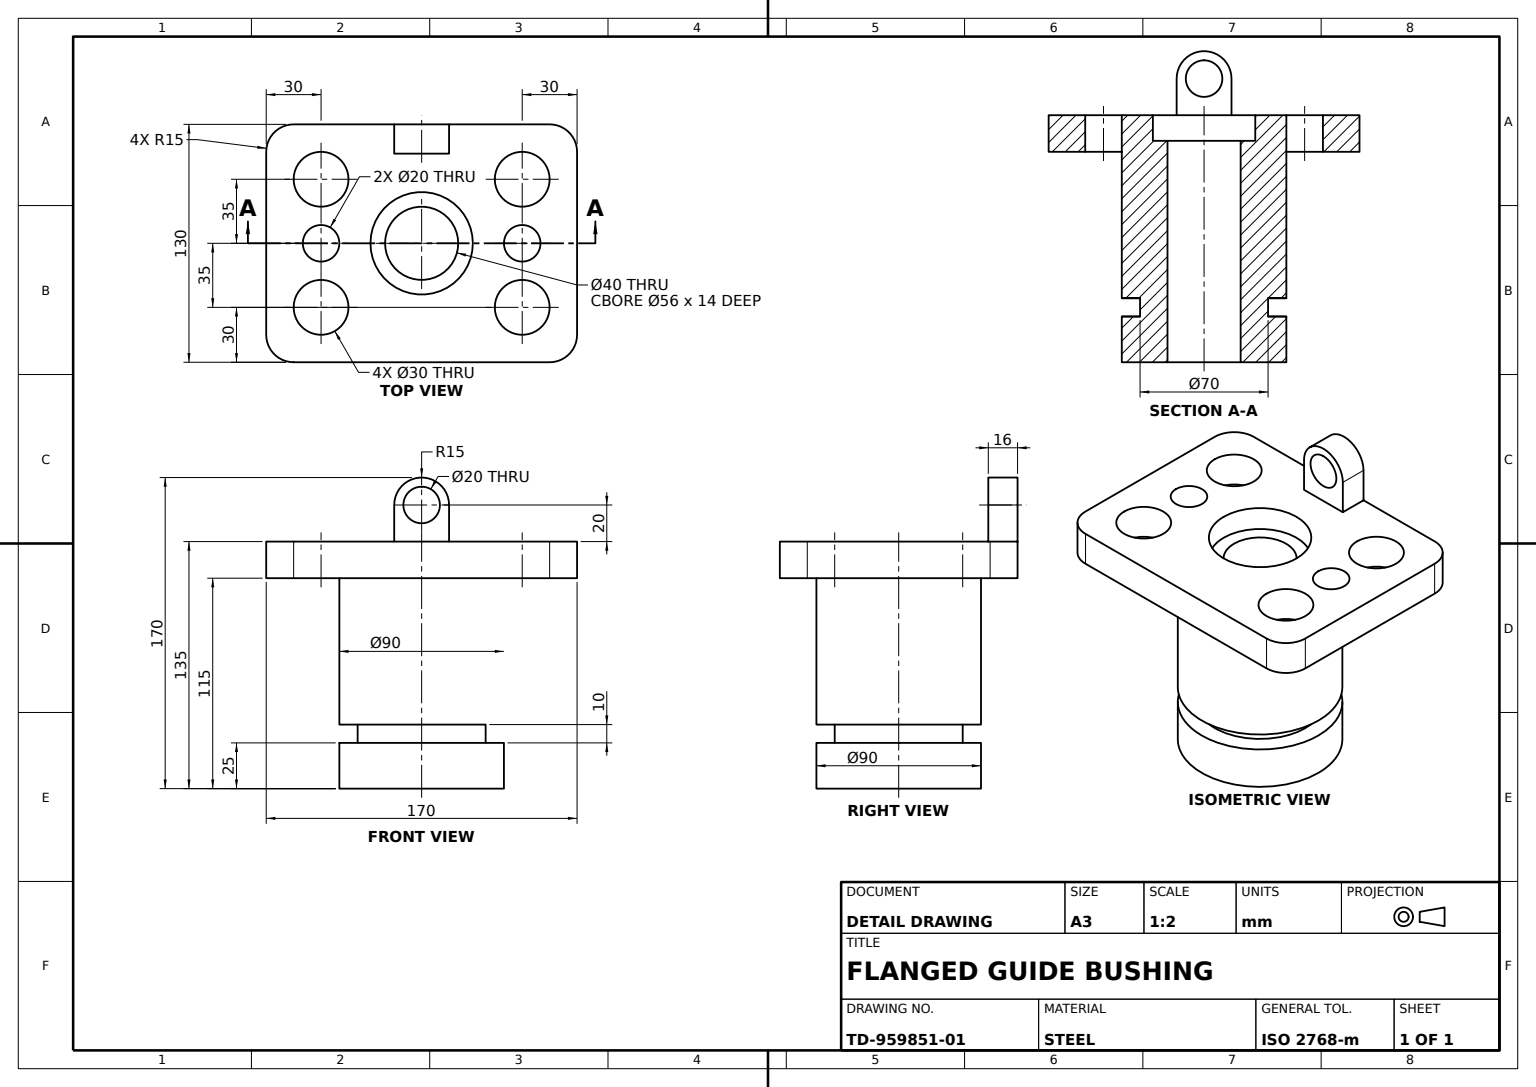
ISO-10303-21;
HEADER;
FILE_DESCRIPTION((''),'2;1');
FILE_NAME('','',(''),(''),'','','');
FILE_SCHEMA(('AUTOMOTIVE_DESIGN'));
ENDSEC;
DATA;
#1=APPLICATION_CONTEXT('');
#2=PRODUCT_CONTEXT('',#1,'mechanical');
#3=PRODUCT('','','',(#2));
#4=PRODUCT_DEFINITION_FORMATION('','',#3);
#5=PRODUCT_DEFINITION_CONTEXT('',#1,'design');
#6=PRODUCT_DEFINITION('','',#4,#5);
#7=PRODUCT_DEFINITION_SHAPE('','',#6);
#8=(LENGTH_UNIT()NAMED_UNIT(*)SI_UNIT(.MILLI.,.METRE.));
#9=(NAMED_UNIT(*)PLANE_ANGLE_UNIT()SI_UNIT($,.RADIAN.));
#10=(NAMED_UNIT(*)SI_UNIT($,.STERADIAN.)SOLID_ANGLE_UNIT());
#11=UNCERTAINTY_MEASURE_WITH_UNIT(LENGTH_MEASURE(0.005),#8,'distance_accuracy_value','');
#12=(GEOMETRIC_REPRESENTATION_CONTEXT(3)GLOBAL_UNCERTAINTY_ASSIGNED_CONTEXT((#11))GLOBAL_UNIT_ASSIGNED_CONTEXT((#8,#9,#10))REPRESENTATION_CONTEXT('',''));
#13=CARTESIAN_POINT('',(-35.,0.,35.));
#14=VERTEX_POINT('',#13);
#15=CARTESIAN_POINT('',(0.,0.,35.));
#16=DIRECTION('',(0.,0.,-1.));
#17=DIRECTION('',(-1.,0.,0.));
#18=AXIS2_PLACEMENT_3D('',#15,#16,#17);
#19=CIRCLE('',#18,35.);
#20=EDGE_CURVE('',#14,#14,#19,.F.);
#21=ORIENTED_EDGE('',*,*,#20,.T.);
#22=EDGE_LOOP('',(#21));
#23=FACE_BOUND('',#22,.T.);
#24=CARTESIAN_POINT('',(-45.,0.,35.));
#25=VERTEX_POINT('',#24);
#26=CIRCLE('',#18,45.);
#27=EDGE_CURVE('',#25,#25,#26,.F.);
#28=ORIENTED_EDGE('',*,*,#27,.F.);
#29=EDGE_LOOP('',(#28));
#30=FACE_BOUND('',#29,.T.);
#31=CARTESIAN_POINT('',(0.,35.,35.));
#32=AXIS2_PLACEMENT_3D('',#31,#16,#17);
#33=PLANE('',#32);
#34=ADVANCED_FACE('',(#23,#30),#33,.T.);
#35=CARTESIAN_POINT('',(45.,0.,115.));
#36=VERTEX_POINT('',#35);
#37=CARTESIAN_POINT('',(55.,0.,115.));
#38=DIRECTION('',(0.,0.,1.));
#39=DIRECTION('',(1.,0.,0.));
#40=AXIS2_PLACEMENT_3D('',#37,#38,#39);
#41=CIRCLE('',#40,10.);
#42=EDGE_CURVE('',#36,#36,#41,.T.);
#43=ORIENTED_EDGE('',*,*,#42,.F.);
#44=EDGE_LOOP('',(#43));
#45=FACE_BOUND('',#44,.T.);
#46=CARTESIAN_POINT('',(45.,0.,135.));
#47=VERTEX_POINT('',#46);
#48=CARTESIAN_POINT('',(55.,0.,135.));
#49=AXIS2_PLACEMENT_3D('',#48,#16,#17);
#50=CIRCLE('',#49,10.);
#51=EDGE_CURVE('',#47,#47,#50,.T.);
#52=ORIENTED_EDGE('',*,*,#51,.F.);
#53=EDGE_LOOP('',(#52));
#54=FACE_BOUND('',#53,.T.);
#55=CYLINDRICAL_SURFACE('',#49,10.);
#56=ADVANCED_FACE('',(#45,#54),#55,.F.);
#57=CARTESIAN_POINT('',(-70.,65.,135.));
#58=VERTEX_POINT('',#57);
#59=CARTESIAN_POINT('',(-85.,50.,135.));
#60=VERTEX_POINT('',#59);
#61=CARTESIAN_POINT('',(-70.,50.,135.));
#62=AXIS2_PLACEMENT_3D('',#61,#38,#39);
#63=CIRCLE('',#62,15.);
#64=EDGE_CURVE('',#58,#60,#63,.T.);
#65=ORIENTED_EDGE('',*,*,#64,.F.);
#66=CARTESIAN_POINT('',(-70.,65.,115.));
#67=VERTEX_POINT('',#66);
#68=VECTOR('',#16,1000.);
#69=LINE('',#57,#68);
#70=EDGE_CURVE('',#67,#58,#69,.F.);
#71=ORIENTED_EDGE('',*,*,#70,.F.);
#72=CARTESIAN_POINT('',(-85.,50.,115.));
#73=VERTEX_POINT('',#72);
#74=CARTESIAN_POINT('',(-70.,50.,115.));
#75=AXIS2_PLACEMENT_3D('',#74,#38,#39);
#76=CIRCLE('',#75,15.);
#77=EDGE_CURVE('',#73,#67,#76,.F.);
#78=ORIENTED_EDGE('',*,*,#77,.F.);
#79=LINE('',#59,#68);
#80=EDGE_CURVE('',#60,#73,#79,.T.);
#81=ORIENTED_EDGE('',*,*,#80,.F.);
#82=EDGE_LOOP('',(#65,#71,#78,#81));
#83=FACE_BOUND('',#82,.T.);
#84=AXIS2_PLACEMENT_3D('',#61,#16,#17);
#85=CYLINDRICAL_SURFACE('',#84,15.);
#86=ADVANCED_FACE('',(#83),#85,.T.);
#87=CARTESIAN_POINT('',(15.,49.,155.));
#88=VERTEX_POINT('',#87);
#89=CARTESIAN_POINT('',(-15.,49.,155.));
#90=VERTEX_POINT('',#89);
#91=CARTESIAN_POINT('',(0.,49.,155.));
#92=DIRECTION('',(0.,-1.,0.));
#93=AXIS2_PLACEMENT_3D('',#91,#92,#39);
#94=CIRCLE('',#93,15.);
#95=EDGE_CURVE('',#88,#90,#94,.T.);
#96=ORIENTED_EDGE('',*,*,#95,.F.);
#97=CARTESIAN_POINT('',(15.,65.,155.));
#98=VERTEX_POINT('',#97);
#99=VECTOR('',#92,1000.);
#100=LINE('',#97,#99);
#101=EDGE_CURVE('',#98,#88,#100,.T.);
#102=ORIENTED_EDGE('',*,*,#101,.F.);
#103=CARTESIAN_POINT('',(-15.,65.,155.));
#104=VERTEX_POINT('',#103);
#105=CARTESIAN_POINT('',(0.,65.,155.));
#106=AXIS2_PLACEMENT_3D('',#105,#92,#39);
#107=CIRCLE('',#106,15.);
#108=EDGE_CURVE('',#98,#104,#107,.T.);
#109=ORIENTED_EDGE('',*,*,#108,.T.);
#110=LINE('',#103,#99);
#111=EDGE_CURVE('',#104,#90,#110,.T.);
#112=ORIENTED_EDGE('',*,*,#111,.T.);
#113=EDGE_LOOP('',(#96,#102,#109,#112));
#114=FACE_BOUND('',#113,.T.);
#115=AXIS2_PLACEMENT_3D('',#105,#92,#16);
#116=CYLINDRICAL_SURFACE('',#115,15.);
#117=ADVANCED_FACE('',(#114),#116,.T.);
#118=CARTESIAN_POINT('',(-70.,-65.,115.));
#119=VERTEX_POINT('',#118);
#120=CARTESIAN_POINT('',(-85.,-50.,115.));
#121=VERTEX_POINT('',#120);
#122=CARTESIAN_POINT('',(-70.,-50.,115.));
#123=AXIS2_PLACEMENT_3D('',#122,#38,#39);
#124=CIRCLE('',#123,15.);
#125=EDGE_CURVE('',#119,#121,#124,.F.);
#126=ORIENTED_EDGE('',*,*,#125,.F.);
#127=CARTESIAN_POINT('',(-70.,-65.,135.));
#128=VERTEX_POINT('',#127);
#129=LINE('',#127,#68);
#130=EDGE_CURVE('',#128,#119,#129,.T.);
#131=ORIENTED_EDGE('',*,*,#130,.F.);
#132=CARTESIAN_POINT('',(-85.,-50.,135.));
#133=VERTEX_POINT('',#132);
#134=CARTESIAN_POINT('',(-70.,-50.,135.));
#135=AXIS2_PLACEMENT_3D('',#134,#38,#39);
#136=CIRCLE('',#135,15.);
#137=EDGE_CURVE('',#133,#128,#136,.T.);
#138=ORIENTED_EDGE('',*,*,#137,.F.);
#139=LINE('',#132,#68);
#140=EDGE_CURVE('',#121,#133,#139,.F.);
#141=ORIENTED_EDGE('',*,*,#140,.F.);
#142=EDGE_LOOP('',(#126,#131,#138,#141));
#143=FACE_BOUND('',#142,.T.);
#144=AXIS2_PLACEMENT_3D('',#134,#16,#17);
#145=CYLINDRICAL_SURFACE('',#144,15.);
#146=ADVANCED_FACE('',(#143),#145,.T.);
#147=CARTESIAN_POINT('',(70.,-65.,135.));
#148=VERTEX_POINT('',#147);
#149=CARTESIAN_POINT('',(-85.,-65.,135.));
#150=VECTOR('',#39,1000.);
#151=LINE('',#149,#150);
#152=EDGE_CURVE('',#128,#148,#151,.T.);
#153=ORIENTED_EDGE('',*,*,#152,.F.);
#154=ORIENTED_EDGE('',*,*,#130,.T.);
#155=CARTESIAN_POINT('',(70.,-65.,115.));
#156=VERTEX_POINT('',#155);
#157=CARTESIAN_POINT('',(-85.,-65.,115.));
#158=LINE('',#157,#150);
#159=EDGE_CURVE('',#119,#156,#158,.T.);
#160=ORIENTED_EDGE('',*,*,#159,.T.);
#161=LINE('',#147,#68);
#162=EDGE_CURVE('',#156,#148,#161,.F.);
#163=ORIENTED_EDGE('',*,*,#162,.T.);
#164=EDGE_LOOP('',(#153,#154,#160,#163));
#165=FACE_BOUND('',#164,.T.);
#166=DIRECTION('',(0.,1.,0.));
#167=AXIS2_PLACEMENT_3D('',#149,#166,#38);
#168=PLANE('',#167);
#169=ADVANCED_FACE('',(#165),#168,.F.);
#170=ORIENTED_EDGE('',*,*,#80,.T.);
#171=CARTESIAN_POINT('',(-85.,65.,115.));
#172=LINE('',#171,#99);
#173=EDGE_CURVE('',#73,#121,#172,.T.);
#174=ORIENTED_EDGE('',*,*,#173,.T.);
#175=ORIENTED_EDGE('',*,*,#140,.T.);
#176=CARTESIAN_POINT('',(-85.,65.,135.));
#177=LINE('',#176,#99);
#178=EDGE_CURVE('',#60,#133,#177,.T.);
#179=ORIENTED_EDGE('',*,*,#178,.F.);
#180=EDGE_LOOP('',(#170,#174,#175,#179));
#181=FACE_BOUND('',#180,.T.);
#182=AXIS2_PLACEMENT_3D('',#176,#39,#16);
#183=PLANE('',#182);
#184=ADVANCED_FACE('',(#181),#183,.F.);
#185=CARTESIAN_POINT('',(-35.,0.,25.));
#186=VERTEX_POINT('',#185);
#187=CARTESIAN_POINT('',(0.,0.,25.));
#188=AXIS2_PLACEMENT_3D('',#187,#16,#17);
#189=CIRCLE('',#188,35.);
#190=EDGE_CURVE('',#186,#186,#189,.F.);
#191=ORIENTED_EDGE('',*,*,#190,.F.);
#192=EDGE_LOOP('',(#191));
#193=FACE_BOUND('',#192,.T.);
#194=CARTESIAN_POINT('',(45.,0.,25.));
#195=VERTEX_POINT('',#194);
#196=AXIS2_PLACEMENT_3D('',#187,#38,#39);
#197=CIRCLE('',#196,45.);
#198=EDGE_CURVE('',#195,#195,#197,.F.);
#199=ORIENTED_EDGE('',*,*,#198,.F.);
#200=EDGE_LOOP('',(#199));
#201=FACE_BOUND('',#200,.T.);
#202=CARTESIAN_POINT('',(0.,45.521823,25.));
#203=AXIS2_PLACEMENT_3D('',#202,#38,#39);
#204=PLANE('',#203);
#205=ADVANCED_FACE('',(#193,#201),#204,.T.);
#206=ORIENTED_EDGE('',*,*,#20,.F.);
#207=EDGE_LOOP('',(#206));
#208=FACE_BOUND('',#207,.T.);
#209=ORIENTED_EDGE('',*,*,#190,.T.);
#210=EDGE_LOOP('',(#209));
#211=FACE_BOUND('',#210,.T.);
#212=CARTESIAN_POINT('',(0.,0.,0.));
#213=AXIS2_PLACEMENT_3D('',#212,#16,#17);
#214=CYLINDRICAL_SURFACE('',#213,35.);
#215=ADVANCED_FACE('',(#208,#211),#214,.T.);
#216=CARTESIAN_POINT('',(-45.,0.,115.));
#217=VERTEX_POINT('',#216);
#218=CARTESIAN_POINT('',(0.,0.,115.));
#219=AXIS2_PLACEMENT_3D('',#218,#38,#39);
#220=CIRCLE('',#219,45.);
#221=EDGE_CURVE('',#36,#217,#220,.T.);
#222=ORIENTED_EDGE('',*,*,#221,.F.);
#223=EDGE_CURVE('',#217,#36,#220,.T.);
#224=ORIENTED_EDGE('',*,*,#223,.F.);
#225=EDGE_LOOP('',(#222,#224));
#226=FACE_BOUND('',#225,.T.);
#227=ORIENTED_EDGE('',*,*,#27,.T.);
#228=EDGE_LOOP('',(#227));
#229=FACE_BOUND('',#228,.T.);
#230=CARTESIAN_POINT('',(0.,0.,135.));
#231=AXIS2_PLACEMENT_3D('',#230,#16,#17);
#232=CYLINDRICAL_SURFACE('',#231,45.);
#233=ADVANCED_FACE('',(#226,#229),#232,.T.);
#234=CARTESIAN_POINT('',(-20.,0.,0.));
#235=VERTEX_POINT('',#234);
#236=CIRCLE('',#213,20.);
#237=EDGE_CURVE('',#235,#235,#236,.T.);
#238=ORIENTED_EDGE('',*,*,#237,.T.);
#239=EDGE_LOOP('',(#238));
#240=FACE_BOUND('',#239,.T.);
#241=CARTESIAN_POINT('',(-20.,0.,121.));
#242=VERTEX_POINT('',#241);
#243=CARTESIAN_POINT('',(0.,0.,121.));
#244=AXIS2_PLACEMENT_3D('',#243,#16,#17);
#245=CIRCLE('',#244,20.);
#246=EDGE_CURVE('',#242,#242,#245,.F.);
#247=ORIENTED_EDGE('',*,*,#246,.T.);
#248=EDGE_LOOP('',(#247));
#249=FACE_BOUND('',#248,.T.);
#250=CARTESIAN_POINT('',(0.,0.,-71.66739));
#251=AXIS2_PLACEMENT_3D('',#250,#16,#17);
#252=CYLINDRICAL_SURFACE('',#251,20.);
#253=ADVANCED_FACE('',(#240,#249),#252,.F.);
#254=CARTESIAN_POINT('',(-15.,65.,135.));
#255=VERTEX_POINT('',#254);
#256=CARTESIAN_POINT('',(-15.,49.,135.));
#257=VERTEX_POINT('',#256);
#258=CARTESIAN_POINT('',(-15.,0.,135.));
#259=LINE('',#258,#99);
#260=EDGE_CURVE('',#255,#257,#259,.T.);
#261=ORIENTED_EDGE('',*,*,#260,.T.);
#262=LINE('',#89,#68);
#263=EDGE_CURVE('',#90,#257,#262,.T.);
#264=ORIENTED_EDGE('',*,*,#263,.F.);
#265=ORIENTED_EDGE('',*,*,#111,.F.);
#266=LINE('',#103,#68);
#267=EDGE_CURVE('',#104,#255,#266,.T.);
#268=ORIENTED_EDGE('',*,*,#267,.T.);
#269=EDGE_LOOP('',(#261,#264,#265,#268));
#270=FACE_BOUND('',#269,.T.);
#271=AXIS2_PLACEMENT_3D('',#103,#17,#38);
#272=PLANE('',#271);
#273=ADVANCED_FACE('',(#270),#272,.T.);
#274=CARTESIAN_POINT('',(15.,49.,135.));
#275=VERTEX_POINT('',#274);
#276=CARTESIAN_POINT('',(15.,49.,122.516247));
#277=VECTOR('',#38,1000.);
#278=LINE('',#276,#277);
#279=EDGE_CURVE('',#275,#88,#278,.T.);
#280=ORIENTED_EDGE('',*,*,#279,.F.);
#281=CARTESIAN_POINT('',(15.,65.,135.));
#282=VERTEX_POINT('',#281);
#283=CARTESIAN_POINT('',(15.,0.,135.));
#284=VECTOR('',#166,1000.);
#285=LINE('',#283,#284);
#286=EDGE_CURVE('',#275,#282,#285,.T.);
#287=ORIENTED_EDGE('',*,*,#286,.T.);
#288=CARTESIAN_POINT('',(15.,65.,122.516247));
#289=LINE('',#288,#277);
#290=EDGE_CURVE('',#282,#98,#289,.T.);
#291=ORIENTED_EDGE('',*,*,#290,.T.);
#292=ORIENTED_EDGE('',*,*,#101,.T.);
#293=EDGE_LOOP('',(#280,#287,#291,#292));
#294=FACE_BOUND('',#293,.T.);
#295=AXIS2_PLACEMENT_3D('',#288,#39,#16);
#296=PLANE('',#295);
#297=ADVANCED_FACE('',(#294),#296,.T.);
#298=CARTESIAN_POINT('',(45.,0.,0.));
#299=VERTEX_POINT('',#298);
#300=AXIS2_PLACEMENT_3D('',#212,#16,#39);
#301=CIRCLE('',#300,45.);
#302=EDGE_CURVE('',#299,#299,#301,.T.);
#303=ORIENTED_EDGE('',*,*,#302,.T.);
#304=EDGE_LOOP('',(#303));
#305=FACE_BOUND('',#304,.T.);
#306=ORIENTED_EDGE('',*,*,#237,.F.);
#307=EDGE_LOOP('',(#306));
#308=FACE_BOUND('',#307,.T.);
#309=PLANE('',#213);
#310=ADVANCED_FACE('',(#305,#308),#309,.T.);
#311=CARTESIAN_POINT('',(-40.,35.,115.));
#312=VERTEX_POINT('',#311);
#313=CARTESIAN_POINT('',(-55.,35.,115.));
#314=AXIS2_PLACEMENT_3D('',#313,#38,#39);
#315=CIRCLE('',#314,15.);
#316=EDGE_CURVE('',#312,#312,#315,.T.);
#317=ORIENTED_EDGE('',*,*,#316,.T.);
#318=EDGE_LOOP('',(#317));
#319=FACE_BOUND('',#318,.T.);
#320=CARTESIAN_POINT('',(-40.,-35.,115.));
#321=VERTEX_POINT('',#320);
#322=CARTESIAN_POINT('',(-55.,-35.,115.));
#323=AXIS2_PLACEMENT_3D('',#322,#38,#39);
#324=CIRCLE('',#323,15.);
#325=EDGE_CURVE('',#321,#321,#324,.T.);
#326=ORIENTED_EDGE('',*,*,#325,.T.);
#327=EDGE_LOOP('',(#326));
#328=FACE_BOUND('',#327,.T.);
#329=CARTESIAN_POINT('',(70.,35.,115.));
#330=VERTEX_POINT('',#329);
#331=CARTESIAN_POINT('',(55.,35.,115.));
#332=AXIS2_PLACEMENT_3D('',#331,#38,#39);
#333=CIRCLE('',#332,15.);
#334=EDGE_CURVE('',#330,#330,#333,.T.);
#335=ORIENTED_EDGE('',*,*,#334,.T.);
#336=EDGE_LOOP('',(#335));
#337=FACE_BOUND('',#336,.T.);
#338=ORIENTED_EDGE('',*,*,#42,.T.);
#339=ORIENTED_EDGE('',*,*,#221,.T.);
#340=CARTESIAN_POINT('',(-55.,0.,115.));
#341=AXIS2_PLACEMENT_3D('',#340,#38,#39);
#342=CIRCLE('',#341,10.);
#343=EDGE_CURVE('',#217,#217,#342,.T.);
#344=ORIENTED_EDGE('',*,*,#343,.T.);
#345=ORIENTED_EDGE('',*,*,#223,.T.);
#346=EDGE_LOOP('',(#338,#339,#344,#345));
#347=FACE_BOUND('',#346,.T.);
#348=CARTESIAN_POINT('',(70.,65.,115.));
#349=VERTEX_POINT('',#348);
#350=CARTESIAN_POINT('',(85.,50.,115.));
#351=VERTEX_POINT('',#350);
#352=CARTESIAN_POINT('',(70.,50.,115.));
#353=AXIS2_PLACEMENT_3D('',#352,#38,#39);
#354=CIRCLE('',#353,15.);
#355=EDGE_CURVE('',#349,#351,#354,.F.);
#356=ORIENTED_EDGE('',*,*,#355,.T.);
#357=CARTESIAN_POINT('',(85.,-50.,115.));
#358=VERTEX_POINT('',#357);
#359=CARTESIAN_POINT('',(85.,-65.,115.));
#360=LINE('',#359,#284);
#361=EDGE_CURVE('',#358,#351,#360,.T.);
#362=ORIENTED_EDGE('',*,*,#361,.F.);
#363=CARTESIAN_POINT('',(70.,-50.,115.));
#364=AXIS2_PLACEMENT_3D('',#363,#38,#39);
#365=CIRCLE('',#364,15.);
#366=EDGE_CURVE('',#358,#156,#365,.F.);
#367=ORIENTED_EDGE('',*,*,#366,.T.);
#368=ORIENTED_EDGE('',*,*,#159,.F.);
#369=ORIENTED_EDGE('',*,*,#125,.T.);
#370=ORIENTED_EDGE('',*,*,#173,.F.);
#371=ORIENTED_EDGE('',*,*,#77,.T.);
#372=CARTESIAN_POINT('',(85.,65.,115.));
#373=VECTOR('',#17,1000.);
#374=LINE('',#372,#373);
#375=EDGE_CURVE('',#349,#67,#374,.T.);
#376=ORIENTED_EDGE('',*,*,#375,.F.);
#377=EDGE_LOOP('',(#356,#362,#367,#368,#369,#370,#371,#376));
#378=FACE_BOUND('',#377,.T.);
#379=CARTESIAN_POINT('',(70.,-35.,115.));
#380=VERTEX_POINT('',#379);
#381=CARTESIAN_POINT('',(55.,-35.,115.));
#382=AXIS2_PLACEMENT_3D('',#381,#38,#39);
#383=CIRCLE('',#382,15.);
#384=EDGE_CURVE('',#380,#380,#383,.T.);
#385=ORIENTED_EDGE('',*,*,#384,.T.);
#386=EDGE_LOOP('',(#385));
#387=FACE_BOUND('',#386,.T.);
#388=PLANE('',#219);
#389=ADVANCED_FACE('',(#319,#328,#337,#347,#378,#387),#388,.F.);
#390=ORIENTED_EDGE('',*,*,#366,.F.);
#391=CARTESIAN_POINT('',(85.,-50.,135.));
#392=VERTEX_POINT('',#391);
#393=LINE('',#391,#68);
#394=EDGE_CURVE('',#392,#358,#393,.T.);
#395=ORIENTED_EDGE('',*,*,#394,.F.);
#396=CARTESIAN_POINT('',(70.,-50.,135.));
#397=AXIS2_PLACEMENT_3D('',#396,#38,#39);
#398=CIRCLE('',#397,15.);
#399=EDGE_CURVE('',#148,#392,#398,.T.);
#400=ORIENTED_EDGE('',*,*,#399,.F.);
#401=ORIENTED_EDGE('',*,*,#162,.F.);
#402=EDGE_LOOP('',(#390,#395,#400,#401));
#403=FACE_BOUND('',#402,.T.);
#404=AXIS2_PLACEMENT_3D('',#396,#16,#17);
#405=CYLINDRICAL_SURFACE('',#404,15.);
#406=ADVANCED_FACE('',(#403),#405,.T.);
#407=CARTESIAN_POINT('',(0.,49.,165.));
#408=VERTEX_POINT('',#407);
#409=AXIS2_PLACEMENT_3D('',#91,#166,#38);
#410=CIRCLE('',#409,10.);
#411=EDGE_CURVE('',#408,#408,#410,.T.);
#412=ORIENTED_EDGE('',*,*,#411,.T.);
#413=EDGE_LOOP('',(#412));
#414=FACE_BOUND('',#413,.T.);
#415=CARTESIAN_POINT('',(0.,49.,135.));
#416=LINE('',#415,#150);
#417=EDGE_CURVE('',#257,#275,#416,.T.);
#418=ORIENTED_EDGE('',*,*,#417,.T.);
#419=ORIENTED_EDGE('',*,*,#279,.T.);
#420=ORIENTED_EDGE('',*,*,#95,.T.);
#421=ORIENTED_EDGE('',*,*,#263,.T.);
#422=EDGE_LOOP('',(#418,#419,#420,#421));
#423=FACE_BOUND('',#422,.T.);
#424=AXIS2_PLACEMENT_3D('',#91,#92,#16);
#425=PLANE('',#424);
#426=ADVANCED_FACE('',(#414,#423),#425,.T.);
#427=CARTESIAN_POINT('',(85.,50.,135.));
#428=VERTEX_POINT('',#427);
#429=LINE('',#427,#68);
#430=EDGE_CURVE('',#351,#428,#429,.F.);
#431=ORIENTED_EDGE('',*,*,#430,.F.);
#432=ORIENTED_EDGE('',*,*,#355,.F.);
#433=CARTESIAN_POINT('',(70.,65.,135.));
#434=VERTEX_POINT('',#433);
#435=LINE('',#433,#68);
#436=EDGE_CURVE('',#434,#349,#435,.T.);
#437=ORIENTED_EDGE('',*,*,#436,.F.);
#438=CARTESIAN_POINT('',(70.,50.,135.));
#439=AXIS2_PLACEMENT_3D('',#438,#38,#39);
#440=CIRCLE('',#439,15.);
#441=EDGE_CURVE('',#428,#434,#440,.T.);
#442=ORIENTED_EDGE('',*,*,#441,.F.);
#443=EDGE_LOOP('',(#431,#432,#437,#442));
#444=FACE_BOUND('',#443,.T.);
#445=AXIS2_PLACEMENT_3D('',#438,#16,#17);
#446=CYLINDRICAL_SURFACE('',#445,15.);
#447=ADVANCED_FACE('',(#444),#446,.T.);
#448=CARTESIAN_POINT('',(-65.,0.,135.));
#449=VERTEX_POINT('',#448);
#450=CARTESIAN_POINT('',(-55.,0.,135.));
#451=AXIS2_PLACEMENT_3D('',#450,#16,#17);
#452=CIRCLE('',#451,10.);
#453=EDGE_CURVE('',#449,#449,#452,.T.);
#454=ORIENTED_EDGE('',*,*,#453,.F.);
#455=EDGE_LOOP('',(#454));
#456=FACE_BOUND('',#455,.T.);
#457=ORIENTED_EDGE('',*,*,#343,.F.);
#458=EDGE_LOOP('',(#457));
#459=FACE_BOUND('',#458,.T.);
#460=CYLINDRICAL_SURFACE('',#451,10.);
#461=ADVANCED_FACE('',(#456,#459),#460,.F.);
#462=ORIENTED_EDGE('',*,*,#325,.F.);
#463=EDGE_LOOP('',(#462));
#464=FACE_BOUND('',#463,.T.);
#465=CARTESIAN_POINT('',(-70.,-35.,135.));
#466=VERTEX_POINT('',#465);
#467=CARTESIAN_POINT('',(-55.,-35.,135.));
#468=AXIS2_PLACEMENT_3D('',#467,#16,#17);
#469=CIRCLE('',#468,15.);
#470=EDGE_CURVE('',#466,#466,#469,.T.);
#471=ORIENTED_EDGE('',*,*,#470,.F.);
#472=EDGE_LOOP('',(#471));
#473=FACE_BOUND('',#472,.T.);
#474=CYLINDRICAL_SURFACE('',#468,15.);
#475=ADVANCED_FACE('',(#464,#473),#474,.F.);
#476=ORIENTED_EDGE('',*,*,#302,.F.);
#477=EDGE_LOOP('',(#476));
#478=FACE_BOUND('',#477,.T.);
#479=ORIENTED_EDGE('',*,*,#198,.T.);
#480=EDGE_LOOP('',(#479));
#481=FACE_BOUND('',#480,.T.);
#482=ADVANCED_FACE('',(#478,#481),#232,.T.);
#483=ORIENTED_EDGE('',*,*,#51,.T.);
#484=EDGE_LOOP('',(#483));
#485=FACE_BOUND('',#484,.T.);
#486=ORIENTED_EDGE('',*,*,#470,.T.);
#487=EDGE_LOOP('',(#486));
#488=FACE_BOUND('',#487,.T.);
#489=CARTESIAN_POINT('',(40.,-35.,135.));
#490=VERTEX_POINT('',#489);
#491=CARTESIAN_POINT('',(55.,-35.,135.));
#492=AXIS2_PLACEMENT_3D('',#491,#16,#17);
#493=CIRCLE('',#492,15.);
#494=EDGE_CURVE('',#490,#490,#493,.T.);
#495=ORIENTED_EDGE('',*,*,#494,.T.);
#496=EDGE_LOOP('',(#495));
#497=FACE_BOUND('',#496,.T.);
#498=CARTESIAN_POINT('',(-28.,0.,135.));
#499=VERTEX_POINT('',#498);
#500=CIRCLE('',#231,28.);
#501=EDGE_CURVE('',#499,#499,#500,.T.);
#502=ORIENTED_EDGE('',*,*,#501,.T.);
#503=EDGE_LOOP('',(#502));
#504=FACE_BOUND('',#503,.T.);
#505=ORIENTED_EDGE('',*,*,#453,.T.);
#506=EDGE_LOOP('',(#505));
#507=FACE_BOUND('',#506,.T.);
#508=CARTESIAN_POINT('',(40.,35.,135.));
#509=VERTEX_POINT('',#508);
#510=CARTESIAN_POINT('',(55.,35.,135.));
#511=AXIS2_PLACEMENT_3D('',#510,#16,#17);
#512=CIRCLE('',#511,15.);
#513=EDGE_CURVE('',#509,#509,#512,.T.);
#514=ORIENTED_EDGE('',*,*,#513,.T.);
#515=EDGE_LOOP('',(#514));
#516=FACE_BOUND('',#515,.T.);
#517=CARTESIAN_POINT('',(-70.,35.,135.));
#518=VERTEX_POINT('',#517);
#519=CARTESIAN_POINT('',(-55.,35.,135.));
#520=AXIS2_PLACEMENT_3D('',#519,#16,#17);
#521=CIRCLE('',#520,15.);
#522=EDGE_CURVE('',#518,#518,#521,.T.);
#523=ORIENTED_EDGE('',*,*,#522,.T.);
#524=EDGE_LOOP('',(#523));
#525=FACE_BOUND('',#524,.T.);
#526=CARTESIAN_POINT('',(85.,-65.,135.));
#527=LINE('',#526,#284);
#528=EDGE_CURVE('',#392,#428,#527,.T.);
#529=ORIENTED_EDGE('',*,*,#528,.T.);
#530=ORIENTED_EDGE('',*,*,#441,.T.);
#531=CARTESIAN_POINT('',(85.,65.,135.));
#532=LINE('',#531,#373);
#533=EDGE_CURVE('',#434,#282,#532,.T.);
#534=ORIENTED_EDGE('',*,*,#533,.T.);
#535=ORIENTED_EDGE('',*,*,#286,.F.);
#536=ORIENTED_EDGE('',*,*,#417,.F.);
#537=ORIENTED_EDGE('',*,*,#260,.F.);
#538=EDGE_CURVE('',#255,#58,#532,.T.);
#539=ORIENTED_EDGE('',*,*,#538,.T.);
#540=ORIENTED_EDGE('',*,*,#64,.T.);
#541=ORIENTED_EDGE('',*,*,#178,.T.);
#542=ORIENTED_EDGE('',*,*,#137,.T.);
#543=ORIENTED_EDGE('',*,*,#152,.T.);
#544=ORIENTED_EDGE('',*,*,#399,.T.);
#545=EDGE_LOOP('',(#529,#530,#534,#535,#536,#537,#539,#540,#541,#542,#543,#544));
#546=FACE_BOUND('',#545,.T.);
#547=AXIS2_PLACEMENT_3D('',#230,#38,#39);
#548=PLANE('',#547);
#549=ADVANCED_FACE('',(#485,#488,#497,#504,#507,#516,#525,#546),#548,.T.);
#550=CARTESIAN_POINT('',(0.,65.,145.));
#551=VERTEX_POINT('',#550);
#552=CIRCLE('',#115,10.);
#553=EDGE_CURVE('',#551,#551,#552,.T.);
#554=ORIENTED_EDGE('',*,*,#553,.T.);
#555=EDGE_LOOP('',(#554));
#556=FACE_BOUND('',#555,.T.);
#557=ORIENTED_EDGE('',*,*,#538,.F.);
#558=ORIENTED_EDGE('',*,*,#267,.F.);
#559=ORIENTED_EDGE('',*,*,#108,.F.);
#560=ORIENTED_EDGE('',*,*,#290,.F.);
#561=ORIENTED_EDGE('',*,*,#533,.F.);
#562=ORIENTED_EDGE('',*,*,#436,.T.);
#563=ORIENTED_EDGE('',*,*,#375,.T.);
#564=ORIENTED_EDGE('',*,*,#70,.T.);
#565=EDGE_LOOP('',(#557,#558,#559,#560,#561,#562,#563,#564));
#566=FACE_BOUND('',#565,.T.);
#567=AXIS2_PLACEMENT_3D('',#531,#92,#16);
#568=PLANE('',#567);
#569=ADVANCED_FACE('',(#556,#566),#568,.F.);
#570=ORIENTED_EDGE('',*,*,#316,.F.);
#571=EDGE_LOOP('',(#570));
#572=FACE_BOUND('',#571,.T.);
#573=ORIENTED_EDGE('',*,*,#522,.F.);
#574=EDGE_LOOP('',(#573));
#575=FACE_BOUND('',#574,.T.);
#576=CYLINDRICAL_SURFACE('',#520,15.);
#577=ADVANCED_FACE('',(#572,#575),#576,.F.);
#578=ORIENTED_EDGE('',*,*,#246,.F.);
#579=EDGE_LOOP('',(#578));
#580=FACE_BOUND('',#579,.T.);
#581=CARTESIAN_POINT('',(-28.,0.,121.));
#582=VERTEX_POINT('',#581);
#583=CIRCLE('',#244,28.);
#584=EDGE_CURVE('',#582,#582,#583,.F.);
#585=ORIENTED_EDGE('',*,*,#584,.T.);
#586=EDGE_LOOP('',(#585));
#587=FACE_BOUND('',#586,.T.);
#588=PLANE('',#244);
#589=ADVANCED_FACE('',(#580,#587),#588,.F.);
#590=ORIENTED_EDGE('',*,*,#334,.F.);
#591=EDGE_LOOP('',(#590));
#592=FACE_BOUND('',#591,.T.);
#593=ORIENTED_EDGE('',*,*,#513,.F.);
#594=EDGE_LOOP('',(#593));
#595=FACE_BOUND('',#594,.T.);
#596=CYLINDRICAL_SURFACE('',#511,15.);
#597=ADVANCED_FACE('',(#592,#595),#596,.F.);
#598=ORIENTED_EDGE('',*,*,#584,.F.);
#599=EDGE_LOOP('',(#598));
#600=FACE_BOUND('',#599,.T.);
#601=ORIENTED_EDGE('',*,*,#501,.F.);
#602=EDGE_LOOP('',(#601));
#603=FACE_BOUND('',#602,.T.);
#604=CYLINDRICAL_SURFACE('',#231,28.);
#605=ADVANCED_FACE('',(#600,#603),#604,.F.);
#606=ORIENTED_EDGE('',*,*,#384,.F.);
#607=EDGE_LOOP('',(#606));
#608=FACE_BOUND('',#607,.T.);
#609=ORIENTED_EDGE('',*,*,#494,.F.);
#610=EDGE_LOOP('',(#609));
#611=FACE_BOUND('',#610,.T.);
#612=CYLINDRICAL_SURFACE('',#492,15.);
#613=ADVANCED_FACE('',(#608,#611),#612,.F.);
#614=ORIENTED_EDGE('',*,*,#411,.F.);
#615=EDGE_LOOP('',(#614));
#616=FACE_BOUND('',#615,.T.);
#617=ORIENTED_EDGE('',*,*,#553,.F.);
#618=EDGE_LOOP('',(#617));
#619=FACE_BOUND('',#618,.T.);
#620=CYLINDRICAL_SURFACE('',#409,10.);
#621=ADVANCED_FACE('',(#616,#619),#620,.F.);
#622=ORIENTED_EDGE('',*,*,#394,.T.);
#623=ORIENTED_EDGE('',*,*,#361,.T.);
#624=ORIENTED_EDGE('',*,*,#430,.T.);
#625=ORIENTED_EDGE('',*,*,#528,.F.);
#626=EDGE_LOOP('',(#622,#623,#624,#625));
#627=FACE_BOUND('',#626,.T.);
#628=AXIS2_PLACEMENT_3D('',#526,#17,#38);
#629=PLANE('',#628);
#630=ADVANCED_FACE('',(#627),#629,.F.);
#631=CLOSED_SHELL('',(#34,#56,#86,#117,#146,#169,#184,#205,#215,#233,#253,#273,#297,#310,#389,#406,#426,#447,#461,#475,#482,#549,#569,#577,#589,#597,#605,#613,#621,#630));
#632=MANIFOLD_SOLID_BREP('',#631);
#633=ADVANCED_BREP_SHAPE_REPRESENTATION('',(#632),#12);
#634=SHAPE_DEFINITION_REPRESENTATION(#7,#633);
ENDSEC;
END-ISO-10303-21;
